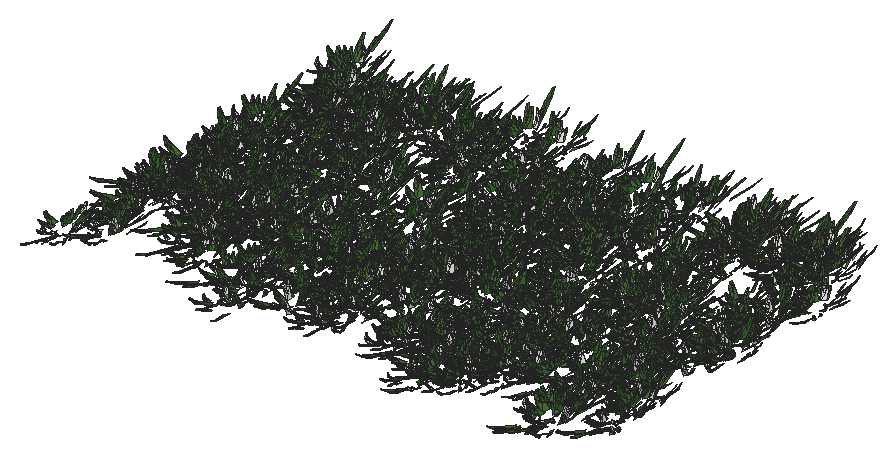
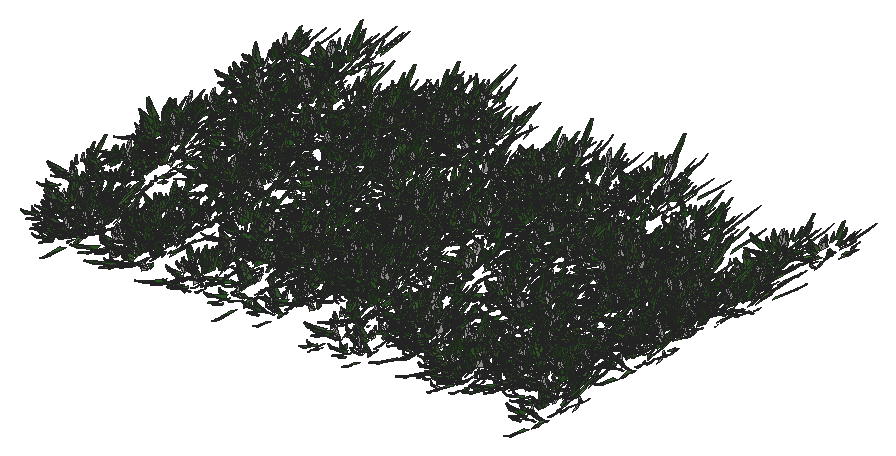
# SketchUp Ruby script. Lengths in inches.
U = 1.inch
M = Sketchup.active_model
def pt(a) = Geom::Point3d.new(a.map { |v| v * U })
def face(e, loops, mat)
  f = e.add_face(loops[0].map { |a| pt(a) })
  loops[1..].each { |l| e.add_face(l.map { |a| pt(a) }).erase! }
  f.material = f.back_material = mat if mat
  f
end
# faces: each face lists its corners as indices into pts; further lists are holes
def faces(e, pts, list, mat = nil) = list.each { |f| face(e, (f[0].is_a?(Array) ? f : [f]).map { |l| l.map { |i| pts[i] } }, mat) }
# xy, xz, yz: faces in a plane at the given z, y or x. An outline is a flat list of corners, or four numbers for a rectangle; further outlines are holes
def ring(l) = l.size == 4 ? [[l[0], l[1]], [l[2], l[1]], [l[2], l[3]], [l[0], l[3]]] : l.each_slice(2).to_a
def flat(e, list, mat, &to3) = list.each { |f| face(e, (f[0].is_a?(Array) ? f : [f]).map { |l| ring(l).map { |u, v| to3.(u, v) } }, mat) }
def xy(e, z, list, mat = nil) = flat(e, list, mat) { |x, y| [x, y, z] }
def xz(e, y, list, mat = nil) = flat(e, list, mat) { |x, z| [x, y, z] }
def yz(e, x, list, mat = nil) = flat(e, list, mat) { |y, z| [x, y, z] }
def lines(e, pts, list) = list.each { |a, b| e.add_line(pt(pts[a]), pt(pts[b])) }
# prism: a flat outline (further loops are holes) pulled along v
def prism(e, loops, v, mat = nil)
  f = face(e, loops, mat); d = Geom::Vector3d.new(v.map { |x| x * U })
  f.pushpull(f.normal.samedirection?(d) ? d.length : -d.length)
end
def box(e, o, s, mat = nil) = prism(e, [[o, [o[0] + s[0], o[1], o[2]], [o[0] + s[0], o[1] + s[1], o[2]], [o[0], o[1] + s[1], o[2]]]], [0, 0, s[2]], mat)
def at(x, y, z, deg = 0) = Geom::Transformation.translation(pt([x, y, z])) * Geom::Transformation.rotation(ORIGIN, Z_AXIS, deg.degrees)
def axes(o, x, y, z) = Geom::Transformation.new([*x, 0, *y, 0, *z, 0, *pt(o).to_a, 1])
def part(name) = M.definitions.add(name)
# library, detail: a bought-in or finely detailed component or shape, given as its bounding box
def library(name, o, s) = part(name).tap { |d| box(d.entities, o, s) }
def detail(e, o, s) = box(e.add_group.entities, o, s)
def put(e, d, t, mat = nil) = e.add_instance(d, t).tap { |i| i.material = mat if mat }
def group(e, t, mat = nil) = e.add_group.tap { |g| g.transformation = t; g.material = mat if mat }.entities
root = M.entities
M.materials.add("Material10").color = [48, 90, 38]
M.materials.add("Material11").color = [68, 110, 48]
M.materials.add("Material12").color = [48, 90, 48]
M.materials.add("Material13").color = [58, 110, 58]
M.materials.add("Material14").color = [58, 90, 38]
M.materials.add("Material15").color = [68, 100, 58]
M.materials.add("Material16").color = [48, 100, 38]
M.materials.add("Material9").color = [68, 110, 58]
c1 = part("grass00")
p = [[-0.6875,0.15,0],[-0.56,0.08,5.52],[-0.04,0.03,2.76],[0.48,-0.02,0],[0.35,-0.02,5.52],[-0.1,-0.14,5.52],
  [-0.12,0.65,8.37],[-0.42,0.65,8.37]]
faces(c1.entities,p,[[0,1,2,3],[3,2,4],[1,5,2],[5,4,2],[1,6,5],[4,5,6],[7,6,1]])
c2 = part("Group16\#1")
put(c2.entities,c1,axes([1.44,-0.61,-0.01],[0.05352,0.12609,0],[-0.10704,0.04543,0.07239],[0.06664,-0.02828,0.11628]),"Material12")
put(c2.entities,c1,axes([0.76,-0.15,-0.01],[0.04676,0.24062,0],[-0.23162,0.04501,0.06642],[0.0652,-0.01267,0.23595]),"Material9")
put(c2.entities,c1,axes([0.79,0.01,-0.01],[-0.00606,0.34651,0],[-0.34381,-0.00602,0.0432],[0.04319,0.00076,0.34386]))
put(c2.entities,c1,axes([1,0.23,-0.01],[-0.07192,0.31144,0],[-0.28722,-0.06632,0.1236],[0.12043,0.02781,0.29478]),"Material11")
put(c2.entities,c1,axes([1.66,0.77,-0.01],[-0.13828,0.29651,0],[-0.21551,-0.1005,0.22471],[0.20365,0.09498,0.23779]),"Material16")
put(c2.entities,c1,axes([0.6875,0.52,-0.01],[-0.18126,0.24051,0],[-0.22746,-0.17142,0.09788],[0.07817,0.05891,0.28481]),"Material11")
put(c2.entities,c1,axes([0.68,0.78,-0.01],[-0.215,0.18688,0],[-0.12385,-0.14248,0.21334],[0.13995,0.16101,0.18878]),"Material9")
put(c2.entities,c1,axes([0.56,1,-0.01],[-0.13756,0.07624,0],[-0.06159,-0.11112,0.0927],[0.04494,0.08108,0.12705]),"Material11")
put(c2.entities,c1,axes([0.2,0.64,-0.01],[-0.23729,0.07254,0],[-0.05711,-0.18681,0.153],[0.04473,0.14632,0.19535]),"Material16")
put(c2.entities,c1,axes([0.0625,0.72,-0.01],[-0.28874,0.02525,0],[-0.02179,-0.24916,0.14647],[0.01276,0.14591,0.25012]),"Material9")
put(c2.entities,c1,axes([-0.08,0.62,-0.01],[-0.34089,-0.04187,0],[0.03255,-0.26504,0.216],[-0.02633,0.21439,0.26703]),"Material16")
put(c2.entities,c1,axes([-0.34,0.98,-0.01],[-0.14314,-0.0493,0],[0.04397,-0.12769,0.06843],[-0.02228,0.0647,0.13505]),"Material16")
put(c2.entities,c1,axes([-0.87,1.45,-0.01],[-0.23488,-0.14114,0],[0.13761,-0.22901,0.06087],[-0.03135,0.05217,0.26717]))
put(c2.entities,c1,axes([-0.72,0.77,-0.01],[-0.14208,-0.13251,0],[0.07209,-0.0773,0.16301],[-0.11118,0.11922,0.1057]),"Material16")
put(c2.entities,c1,axes([-0.62,0.43,-0.01],[-0.14845,-0.21203,0],[0.18654,-0.13061,0.12304],[-0.10079,0.07057,0.22772]),"Material9")
put(c2.entities,c1,axes([-0.68,0.29,-0.01],[-0.13639,-0.32136,0],[0.31723,-0.13464,0.05579],[-0.05136,0.0218,0.34462]),"Material10")
put(c2.entities,c1,axes([-0.64,0.125,-0.01],[-0.0458,-0.23569,0],[0.22124,-0.043,0.08276],[-0.08124,0.01579,0.22538]),"Material13")
put(c2.entities,c1,axes([-1.6,-0.03,-0.01],[0.00576,-0.32897,0],[0.27526,0.00482,0.18018],[-0.18015,-0.00315,0.2753]),"Material11")
put(c2.entities,c1,axes([-1.36,-0.31,-0.01],[0.05718,-0.24765,0],[0.18172,0.04196,0.17267],[-0.16825,-0.03885,0.1865]),"Material16")
put(c2.entities,c1,axes([-1.54,-0.72,-0.01],[0.06537,-0.14017,0],[0.13555,0.06321,0.03939],[-0.0357,-0.01665,0.14956]))
put(c2.entities,c1,axes([-1.19,-0.9,-0.01],[0.09597,-0.12735,0],[0.11214,0.08451,0.07557],[-0.06035,-0.04548,0.14042]),"Material15")
put(c2.entities,c1,axes([-0.47,-0.54,-0.01],[0.11588,-0.10072,0],[0.0618,0.0711,0.12124],[-0.07953,-0.0915,0.0942]))
put(c2.entities,c1,axes([-0.47,-0.84,-0.01],[0.11927,-0.0661,0],[0.06603,0.11913,0.00646],[-0.00313,-0.00565,0.13621]),"Material11")
put(c2.entities,c1,axes([-0.38,-1.24,-0.01],[0.28037,-0.08571,0],[0.0618,0.20215,0.20315],[-0.05939,-0.19428,0.21139]),"Material15")
put(c2.entities,c1,axes([-0.06,-0.66,-0.01],[0.22719,-0.01987,0],[0.01247,0.14255,0.17758],[-0.01547,-0.17691,0.1431]),"Material14")
put(c2.entities,c1,axes([0.11,-0.89,-0.01],[0.14882,0.01828,0],[-0.01058,0.08611,0.12229],[0.01491,-0.12138,0.08676]),"Material12")
put(c2.entities,c1,axes([0.25,-0.72,-0.01],[0.20481,0.07053,0],[-0.06206,0.18022,0.10291],[0.03351,-0.0973,0.1906]),"Material12")
put(c2.entities,c1,axes([0.85,-1.42,-0.01],[0.16481,0.09904,0],[-0.09472,0.15762,0.05616],[0.02893,-0.04814,0.18389]),"Material11")
put(c2.entities,c1,axes([1.01,-1.09,-0.01],[0.21858,0.20385,0],[-0.17495,0.1876,0.15339],[0.10462,-0.11218,0.25652]),"Material16")
put(c2.entities,c1,axes([1.01,-0.71,-0.01],[0.08733,0.12473,0],[-0.06445,0.04512,0.13037],[0.1068,-0.07477,0.07867]),"Material12")
c3 = part("Group15\#1")
put(c3.entities,c2,at(0,0,0))
c4 = part("3darcstudiotree_grass00\#1")
put(c4.entities,c3,at(0,0,0))
put(root,c4,axes([800.04,262.41,12.99],[2.7,0,0],[0,6.17186,0],[0,0,1]))
put(root,c4,axes([917.3,263.62,12.99],[2.38747,-5.84405,0],[1.86441,3.9799,-0.01281],[0.0419,0.08945,1.56626]))
put(root,c4,axes([963.49,263.61,12.99],[3.1855,-0.69888,0],[0.31577,7.52063,-0.01064],[0.00398,0.0948,1.77558]))
put(root,c4,axes([857.27,263.68,12.99],[0.83355,-7.41561,0],[3.09264,1.81642,-0.01129],[0.04659,0.02737,1.86628]))
put(root,c4,axes([923.31,262.57,12.99],[0.33488,7.26637,0],[-2.49247,0.60022,-0.01763],[-0.08203,0.01975,1.60818]))
put(root,c4,axes([959.86,263.95,12.99],[1.44327,6.89971,0],[-2.84,3.10412,-0.01048],[-0.03086,0.03373,1.40926]))
put(root,c4,axes([930.6875,263.82,12.99],[-1.38125,4.89434,0],[-2.32777,-3.43262,-0.00439],[-0.01618,-0.02386,1.66469]))
put(root,c4,axes([809.18,269.67,12.99],[2.32785,-1.7688,0],[0.90077,6.19434,-0.00205],[0.00297,0.0204,1.79239]))
put(root,c4,axes([927.87,269.13,12.99],[1.92436,4.50414,0],[-1.90906,4.26186,-0.01838],[-0.05956,0.13295,1.65818]))
put(root,c4,axes([881,271.05,12.99],[1.20789,-7.06216,0],[2.40185,2.14654,-0.00888],[0.04378,0.03913,1.87213]))
put(root,c4,axes([917.85,271.49,12.99],[2.32526,-3.29254,0],[1.36916,5.0524,-0.00486],[0.01024,0.03779,1.42853]))
put(root,c4,axes([904.81,269.45,12.99],[-0.10545,5.83441,0],[-3.03207,-0.28635,-0.00296],[-0.01053,-0.00099,1.47961]))
put(root,c4,axes([848.52,270.28,12.99],[-2.86781,-2.90219,0],[1.05587,-5.45181,-0.0129],[0.01926,-0.09946,1.31952]))
put(root,c4,axes([870.9,270,12.99],[-2.52758,-1.38361,0],[0.5978,-5.70627,-0.00326],[0.00418,-0.03989,1.93944]))
put(root,c4,axes([857.84,271.55,12.99],[2.23594,4.22907,0],[-2.10254,5.80848,-0.00662],[-0.01529,0.04223,1.63949]))
put(root,c4,axes([975.87,271.71,12.99],[-2.17015,-3.00979,0],[1.54385,-5.81652,-0.00574],[0.00982,-0.03699,1.3472]))
put(root,c4,axes([886.64,271.69,12.99],[-3.01605,-0.65305,0],[0.2537,-6.12235,-0.02721],[0.00917,-0.22119,1.31849]))
put(root,c4,axes([930.11,272.08,12.99],[-0.07823,6.60785,0],[-2.80866,-0.17375,-0.00627],[-0.0264,-0.00163,1.62459]))
put(root,c4,axes([837.41,273.87,12.99],[2.08169,2.96658,0],[-1.3434,4.92572,-0.0044],[-0.00874,0.03206,1.30779]))
put(root,c4,axes([908.97,273.63,12.99],[-1.89759,-3.75446,0],[2.03916,-5.38532,-0.00422],[0.0086,-0.02272,1.33295]))
put(root,c4,axes([937.6,272.88,12.99],[-2.04959,5.39493,0],[-1.93192,-3.83508,-0.01448],[-0.04359,-0.08654,1.39954]))
put(root,c4,axes([905.67,278.18,12.99],[2.72294,1.91373,0],[-0.9507,7.06818,-0.02064],[-0.0201,0.1494,1.46981]))
put(root,c4,axes([829.02,279.77,12.99],[3.08767,-0.14916,0],[0.073,7.89587,-0.00824],[0.00059,0.06356,1.59977]))
put(root,c4,axes([958.97,279.01,12.99],[2.42942,0.9007,0],[-0.3986,5.61781,-0.01255],[-0.00963,0.13565,1.63564]))
put(root,c4,axes([918.12,279.84,12.99],[1.13155,-6.43414,0],[3.10428,2.85266,-0.01772],[0.06404,0.05885,1.7874]))
put(root,c4,axes([880.3125,277.63,12.99],[-0.75225,6.31697,0],[-3.37261,-2.09857,-0.0223],[-0.07136,-0.0444,1.58974]))
put(root,c4,axes([962.21,281.1,12.99],[2.38111,-3.79736,0],[1.53061,5.01498,-0.00731],[0.02053,0.06727,1.80073]))
put(root,c4,axes([849.95,278.59,12.99],[0.34869,6.4109,0],[-2.60714,0.74096,-0.00588],[-0.02211,0.00628,1.36568]))
put(root,c4,axes([885.77,281.27,12.99],[0.7386,-7.32123,0],[2.79869,1.47532,-0.00305],[0.01335,0.00704,1.76865]))
put(root,c4,axes([935.57,282.06,12.99],[2.75603,-0.4722,0],[0.25779,7.86192,-0.00347],[0.00106,0.03225,1.92949]))
put(root,c4,axes([910.36,280.67,12.99],[-1.15582,-5.1991,0],[2.69556,-3.13124,-0.00876],[0.02742,-0.03185,1.45672]))
put(root,c4,axes([942.89,280.23,12.99],[-2.27003,3.99727,0],[-1.65257,-4.9038,-0.00087],[-0.0024,-0.00712,1.68429]))
put(root,c4,axes([948.56,280.99,12.99],[-0.12493,7.61806,0],[-3.19755,-0.27399,-0.00219],[-0.00695,-0.0006,1.39308]))
put(root,c4,axes([975.82,281.26,12.99],[0.2055,7.05815,0],[-2.85108,0.43374,-0.01024],[-0.04748,0.00722,1.82096]))
put(root,c4,axes([931.78,281.15,12.99],[-2.67022,3.47951,0],[-1.66016,-6.65707,-0.01918],[-0.03722,-0.14925,1.80194]))
put(root,c4,axes([832.71,281.82,12.99],[-0.53511,7.34039,0],[-2.42448,-0.92353,-0.00349],[-0.01382,-0.00526,1.35435]))
put(root,c4,axes([860.4,282.61,12.99],[0.72731,6.87217,0],[-3.18797,1.76298,-0.01063],[-0.03416,0.01889,1.48723]))
put(root,c4,axes([896.94,284.16,12.99],[1.87008,4.14786,0],[-1.74039,4.10002,-0.00683],[-0.02423,0.05708,1.74693]))
put(root,c4,axes([923.78,283.13,12.99],[-2.48601,3.66419,0],[-1.4306,-5.07163,-0.01497],[-0.03275,-0.1161,1.4615]))
put(root,c4,axes([807.91,283.51,12.99],[-2.35772,1.35875,0],[-0.81657,-7.40372,-0.01943],[-0.01386,-0.12571,1.33771]))
put(root,c4,axes([874.16,286.77,12.99],[-0.61646,-6.32739,0],[2.39607,-1.2198,-0.00779],[0.03137,-0.01597,1.38852]))
put(root,c4,axes([877.7,287.98,12.99],[0.64081,-7.01541,0],[3.23891,1.5459,-0.01659],[0.05554,0.02651,1.55232]))
put(root,c4,axes([934.12,286.84,12.99],[-2.22659,-5.00524,0],[1.72181,-4.00226,-0.00764],[0.02885,-0.06706,1.81511]))
put(root,c4,axes([970.36,288.42,12.99],[2.84331,-3.25189,0],[1.12434,5.13679,-0.01525],[0.03164,0.14454,1.59832]))
put(root,c4,axes([866.375,287.55,12.99],[2.09267,4.86523,0],[-2.41334,5.424,-0.00938],[-0.02819,0.06335,1.95578]))
put(root,c4,axes([860.99,287.44,12.99],[1.71454,5.32814,0],[-2.62121,4.40736,-0.02079],[-0.05084,0.08548,1.35493]))
put(root,c4,axes([832.58,287.21,12.99],[-2.92579,-1.11429,0],[0.42132,-5.78045,-0.01531],[0.01289,-0.17687,1.80136]))
put(root,c4,axes([954.84,288.45,12.99],[2.5236,5.2118,0],[-1.70252,4.30755,-0.00582],[-0.01752,0.04433,1.56404]))
put(root,c4,axes([881.48,287.16,12.99],[-1.22954,6.26972,0],[-3.05141,-3.12679,-0.00369],[-0.01159,-0.01187,1.57624]))
put(root,c4,axes([804.26,288.01,12.99],[-2.71738,0.38743,0],[-0.21027,-7.70598,-0.0193],[-0.00346,-0.12694,1.33558]))
put(root,c4,axes([822.86,289.17,12.99],[-2.58469,-3.57399,0],[1.81595,-6.86221,-0.00291],[0.00482,-0.01821,1.54121]))
put(root,c4,axes([892.49,290.6,12.99],[-2.06789,-3.5248,0],[1.77407,-5.43836,-0.00029],[0.00072,-0.00221,1.69542]))
put(root,c4,axes([962.21,293.48,12.99],[2.12983,-3.59469,0],[1.82781,5.65873,-0.02283],[0.04662,0.14433,1.4512]))
put(root,c4,axes([915.64,293.58,12.99],[-2.48939,1.64634,0],[-0.90667,-7.16359,-0.00573],[-0.00569,-0.04497,1.59925]))
put(root,c4,axes([849.78,296.35,12.99],[3.03864,2.23289,0],[-0.83228,5.91815,-0.00634],[-0.00906,0.06441,1.74238]))
put(root,c4,axes([840.73,297.52,12.99],[1.03012,-7.4017,0],[3.23958,2.35585,-0.00448],[0.01639,0.01192,1.79011]))
put(root,c4,axes([837.5,297.42,12.99],[2.43111,3.00661,0],[-1.55779,6.58177,-0.00222],[-0.00378,0.01596,1.6055]))
put(root,c4,axes([942.25,297.23,12.99],[2.57694,4.09984,0],[-1.65293,5.42872,-0.01513],[-0.03119,0.10243,1.43215]))
put(root,c4,axes([821.38,299.23,12.99],[1.07572,-5.84235,0],[2.48393,2.38976,-0.00467],[0.01652,0.01589,1.41828]))
put(root,c4,axes([927.02,299.19,12.99],[0.86437,-6.35811,0],[2.8703,2.03893,-0.02169],[0.07747,0.05503,1.54236]))
put(root,c4,axes([966.95,296.75,12.99],[-2.417,-2.20097,0],[1.23575,-7.09086,-0.00121],[0.00188,-0.01079,1.92636]))
put(root,c4,axes([960.58,300.01,12.99],[2.78311,-1.49092,0],[0.79705,7.77445,-0.02268],[0.0167,0.16291,1.5468]))
put(root,c4,axes([803.91,296.6,12.99],[-1.85614,4.7772,0],[-2.25295,-4.57397,-0.01682],[-0.04757,-0.09658,1.56312]))
put(root,c4,axes([800.78,298.2,12.99],[-3.39513,-1.95103,0],[0.6221,-5.65666,-0.02201],[0.02063,-0.18756,1.34565]))
put(root,c4,axes([844.1875,300.62,12.99],[0.42428,-7.25386,0],[3.26573,0.99808,-0.0102],[0.03957,0.01209,1.76846]))
put(root,c4,axes([869.55,300.12,12.99],[-0.38453,-6.31098,0],[2.66942,-0.84987,-0.01078],[0.05195,-0.01654,1.79898]))
put(root,c4,axes([823.7,298.59,12.99],[0.52039,6.35,0],[-3.21501,1.37671,-0.00799],[-0.02639,0.0113,1.50733]))
put(root,c4,axes([816.67,298.56,12.99],[-1.20671,7.00574,0],[-2.5747,-2.3173,-0.00571],[-0.02552,-0.02297,1.8245]))
put(root,c4,axes([939.32,298.34,12.99],[-2.52179,3.319,0],[-1.73482,-6.8875,-0.0199],[-0.03481,-0.13822,1.67187]))
put(root,c4,axes([832.82,302.06,12.99],[2.17019,-5.0615,0],[2.038,4.5659,-0.0131],[0.04299,0.09632,1.79861]))
put(root,c4,axes([872.15,299.41,12.99],[-0.72304,6.51011,0],[-2.8107,-1.63115,-0.01715],[-0.061,-0.0354,1.46021]))
put(root,c4,axes([946.49,302.58,12.99],[0.31883,-7.14557,0],[2.92003,0.6808,-0.00761],[0.0365,0.00851,1.94156]))
put(root,c4,axes([807.33,299.89,12.99],[-3.25155,-0.36081,0],[0.16309,-7.67994,-0.01036],[0.00152,-0.07171,1.39846]))
put(root,c4,axes([930.53,303.07,12.99],[0.15852,-7.06641,0],[2.67457,0.31351,-0.01161],[0.04564,0.00535,1.44612]))
put(root,c4,axes([852.04,300.82,12.99],[-2.59908,2.50883,0],[-1.30475,-7.06283,-0.01449],[-0.02018,-0.10921,1.64714]))
put(root,c4,axes([878.57,302.51,12.99],[1.97562,5.89767,0],[-2.42977,4.25298,-0.02004],[-0.05173,0.09056,1.3651]))
put(root,c4,axes([909.24,302.49,12.99],[1.5456,5.93648,0],[-2.54028,3.45586,-0.00188],[-0.0075,0.01021,1.87843]))
put(root,c4,axes([923.3,303.05,12.99],[-1.79443,-4.99456,0],[2.00974,-3.77289,-0.021],[0.06382,-0.11982,1.40308]))
put(root,c4,axes([859.74,303.09,12.99],[-2.02561,-3.51282,0],[1.54104,-4.64322,-0.01586],[0.04171,-0.12567,1.52204]))
put(root,c4,axes([864.36,301.8,12.99],[-1.83508,5.30373,0],[-1.98024,-3.58012,-0.01059],[-0.03213,-0.05808,1.33934]))
put(root,c4,axes([895.01,301.85,12.99],[-2.19701,4.95047,0],[-2.33123,-5.40599,-0.01243],[-0.03382,-0.07843,1.76595]))
put(root,c4,axes([832.47,305.51,12.99],[0.69474,-6.92422,0],[2.54124,1.3323,-0.013],[0.06964,0.03651,1.96601]))
put(root,c4,axes([810.88,306.875,12.99],[1.4124,-5.84324,0],[2.17134,2.74244,-0.00396],[0.01979,0.025,1.94458]))
put(root,c4,axes([924.08,306.78,12.99],[2.8247,4.73688,0],[-1.75886,5.48043,-0.00415],[-0.00798,0.02486,1.32509]))
put(root,c4,axes([958.39,307.92,12.99],[0.18918,-5.93725,0],[2.46344,0.41016,-0.00937],[0.05346,0.0089,1.93766]))
put(root,c4,axes([943.66,307.45,12.99],[-0.98178,-5.4385,0],[3.04457,-2.87189,-0.01762],[0.05342,-0.05039,1.48208]))
put(root,c4,axes([889.55,307.28,12.99],[2.53566,4.2535,0],[-1.4585,4.54314,-0.01519],[-0.03587,0.11174,1.34969]))
put(root,c4,axes([825.69,307.64,12.99],[-2.2701,-5.60069,0],[2.40685,-5.0975,-0.02123],[0.0498,-0.10548,1.43939]))
put(root,c4,axes([930.18,307.26,12.99],[-2.36351,-2.23042,0],[0.9748,-5.3975,-0.01181],[0.0223,-0.12346,1.73426]))
put(root,c4,axes([821.16,306.41,12.99],[-2.92117,0.05351,0],[-0.02548,-7.26875,-0.00779],[-0.00024,-0.06979,1.71052]))
put(root,c4,axes([878.84,309.875,12.99],[2.04745,-6.51457,0],[2.11012,3.46529,-0.0087],[0.03185,0.0523,1.60603]))
put(root,c4,axes([914.72,307.3,12.99],[-2.93231,-1.1271,0],[0.47714,-6.48628,-0.0114],[0.00945,-0.12852,1.97478]))
put(root,c4,axes([880.41,307.71,12.99],[-3.04145,2.20175,0],[-0.83651,-6.03796,-0.01419],[-0.01972,-0.14237,1.75006]))
put(root,c4,axes([954.95,310.73,12.99],[2.62032,1.70998,0],[-0.88973,7.12409,-0.00872],[-0.00816,0.06535,1.51538]))
put(root,c4,axes([898.8,311.28,12.99],[0.93532,-6.17742,0],[2.31038,1.82785,-0.00044],[0.00165,0.00131,1.32507]))
put(root,c4,axes([892.47,309.53,12.99],[1.93534,5.53987,0],[-1.92573,3.51525,-0.01421],[-0.04631,0.08453,1.40932]))
put(root,c4,axes([839.58,307.94,12.99],[-2.73946,3.39326,0],[-1.63174,-6.88341,-0.0133],[-0.02626,-0.11077,1.94738]))
put(root,c4,axes([903.11,308.83,12.99],[-2.55398,0.81074,0],[-0.4474,-7.36433,-0.02154],[-0.00952,-0.15675,1.4342]))
put(root,c4,axes([808.54,311.97,12.99],[0.7552,-6.08854,0],[2.38927,1.54853,-0.01712],[0.0682,0.0442,1.41054]))
put(root,c4,axes([803.77,311.92,12.99],[3.3266,0.63895,0],[-0.23828,6.48218,-0.00911],[-0.00381,0.10354,1.94776]))
put(root,c4,axes([972.21,310.24,12.99],[-3.08545,-0.82643,0],[0.29814,-5.8162,-0.00847],[0.00513,-0.09999,1.82708]))
put(root,c4,axes([851.83,311.58,12.99],[-3.08185,-0.89983,0],[0.3691,-6.60553,-0.0157],[0.0096,-0.17185,1.92971]))
put(root,c4,axes([898.52,316.46,12.99],[2.51781,1.40451,0],[-0.60275,5.64605,-0.01459],[-0.01741,0.16312,1.75568]))
put(root,c4,axes([857.03,317.29,12.99],[0.97248,-5.43024,0],[2.74843,2.57188,-0.00546],[0.01653,0.01547,1.33158]))
put(root,c4,axes([820.46,317.02,12.99],[-0.67912,-5.50704,0],[3.32319,-2.14134,-0.01485],[0.05445,-0.03509,1.80381]))
put(root,c4,axes([902.66,315.91,12.99],[0.99029,6.51274,0],[-2.34145,1.86032,-0.01128],[-0.057,0.04529,1.81963]))
put(root,c4,axes([955.89,316.01,12.99],[-3.28824,0.13443,0],[-0.05478,-7.00185,-0.01042],[-0.00081,-0.10317,1.82123]))
put(root,c4,axes([882.99,319.04,12.99],[0.62571,-7.4238,0],[2.94441,1.29673,-0.00212],[0.0084,0.0037,1.6588]))
put(root,c4,axes([892.45,318,12.99],[-2.53583,-4.0256,0],[1.48452,-4.88632,-0.00375],[0.01093,-0.03599,1.82358]))
put(root,c4,axes([868.75,320.79,12.99],[2.77706,0.31623,0],[-0.16258,7.46024,-0.00527],[-0.00093,0.04278,1.59512]))
put(root,c4,axes([888.66,318.73,12.99],[0.80267,7.165,0],[-3.15194,1.84504,-0.00469],[-0.01633,0.00956,1.60422]))
put(root,c4,axes([977.2,318.72,12.99],[-2.91667,0.89835,0],[-0.39992,-6.78455,-0.01091],[-0.00661,-0.11222,1.8656]))
put(root,c4,axes([829.32,318.99,12.99],[-2.18033,3.33173,0],[-1.37245,-4.69302,-0.00767],[-0.02058,-0.07038,1.63569]))
put(root,c4,axes([805.42,320.86,12.99],[1.14348,5.78612,0],[-2.65712,2.74382,-0.01637],[-0.05127,0.05294,1.37485]))
put(root,c4,axes([942.13,321.15,12.99],[1.19769,4.92215,0],[-2.15095,2.7348,-0.00131],[-0.00659,0.00838,1.9458]))
put(root,c4,axes([810.95,320.35,12.99],[-2.92732,3.88004,0],[-1.36061,-5.36382,-0.01457],[-0.02627,-0.10357,1.33777]))
put(root,c4,axes([898.36,324.18,12.99],[0.03291,-6.00432,0],[2.63901,0.07558,-0.00992],[0.0362,0.00104,1.32167]))
put(root,c4,axes([923.375,321.65,12.99],[-3.18224,0.86052,0],[-0.37285,-7.20456,-0.02284],[-0.00893,-0.17251,1.44864]))
put(root,c4,axes([812.33,325.94,12.99],[3.02492,0.43164,0],[-0.19956,7.30757,-0.00965],[-0.00215,0.07872,1.57035]))
put(root,c4,axes([915.71,325.16,12.99],[-1.84468,-5.41874,0],[2.11551,-3.76307,-0.01663],[0.06746,-0.12,1.89037]))
put(root,c4,axes([974.43,325.54,12.99],[-1.74487,-6.43859,0],[2.07818,-2.9428,-0.00146],[0.0049,-0.00694,1.32424]))
put(root,c4,axes([967.55,327.01,12.99],[1.10448,-5.04762,0],[2.62608,3.00251,-0.01805],[0.06349,0.07259,1.58457]))
put(root,c4,axes([822.98,327.14,12.99],[0.73177,-6.13131,0],[2.98154,1.85938,-0.01691],[0.06168,0.03847,1.6028]))
put(root,c4,axes([952.48,327.69,12.99],[2.63854,-1.95158,0],[0.97491,6.88724,-0.01717],[0.0181,0.12789,1.48777]))
put(root,c4,axes([805.25,324.39,12.99],[-2.42706,4.93315,0],[-1.99413,-5.12641,-0.01814],[-0.05083,-0.13068,1.73642]))
put(root,c4,axes([971.81,324.9,12.99],[-2.78825,0.16165,0],[-0.07676,-6.91806,-0.00196],[-0.00018,-0.01617,1.49745]))
put(root,c4,axes([809.46,328.08,12.99],[2.95238,2.58076,0],[-1.15167,6.88427,-0.01506],[-0.01861,0.11123,1.52965]))
put(root,c4,axes([944.32,328.5,12.99],[2.61895,-0.43156,0],[0.18005,5.70926,-0.00836],[0.00346,0.10957,1.97523]))
put(root,c4,axes([837.86,328.27,12.99],[2.46316,1.62969,0],[-0.82342,6.50301,-0.02015],[-0.02259,0.17839,1.63787]))
put(root,c4,axes([852.25,328.88,12.99],[2.85427,2.32984,0],[-1.05964,6.78315,-0.00059],[-0.0008,0.00513,1.74794]))
put(root,c4,axes([938.04,326.12,12.99],[-2.27649,5.59218,0],[-2.46107,-5.23495,-0.01383],[-0.03262,-0.06938,1.48532]))
put(root,c4,axes([865.68,330.02,12.99],[2.66505,-1.9717,0],[0.98856,6.98188,-0.01611],[0.01782,0.12585,1.58139]))
put(root,c4,axes([843.36,327.72,12.99],[-2.36277,-1.95854,0],[0.89847,-5.66367,-0.00444],[0.00582,-0.03672,1.39182]))
put(root,c4,axes([936.27,327.97,12.99],[0.32715,6.23275,0],[-2.51704,0.69035,-0.01784],[-0.09179,0.02517,1.80168]))
put(root,c4,axes([917.54,328.21,12.99],[0.12673,7.92084,0],[-3.40439,0.28461,-0.0182],[-0.05632,0.00471,1.44668]))
put(root,c4,axes([948.17,330.9,12.99],[-0.57245,-6.81875,0],[2.52981,-1.10975,-0.00431],[0.01615,-0.00708,1.34772]))
put(root,c4,axes([828.03,328.59,12.99],[-1.27604,6.78841,0],[-2.45183,-2.4082,-0.02574],[-0.08568,-0.08415,1.32606]))
put(root,c4,axes([882.02,329.15,12.99],[-2.46614,5.52221,0],[-1.73214,-4.04198,-0.00183],[-0.0053,-0.01236,1.40539]))
put(root,c4,axes([889.25,333.54,12.99],[0.3601,-5.92996,0],[2.68874,0.85315,-0.0013],[0.00642,0.00204,1.85519]))
put(root,c4,axes([848.86,335.1,12.99],[1.7227,-4.93277,0],[1.96338,3.58283,-0.01018],[0.03495,0.06377,1.51436]))
put(root,c4,axes([840.65,336.51,12.99],[2.99045,1.2301,0],[-0.61695,7.83693,-0.01866],[-0.01187,0.15082,1.717]))
put(root,c4,axes([820.88,337.89,12.99],[1.96108,-4.17941,0],[2.3724,5.81667,-0.02398],[0.04727,0.11591,1.37951]))
put(root,c4,axes([898.62,337.12,12.99],[2.6618,2.65939,0],[-1.14151,5.97005,-0.01451],[-0.02379,0.1244,1.59989]))
put(root,c4,axes([893.15,338.71,12.99],[3.14408,2.86339,0],[-1.15655,6.63566,-0.01606],[-0.02146,0.12312,1.54782]))
put(root,c4,axes([812.29,339.55,12.99],[2.36646,-1.30514,0],[0.68088,6.45085,-0.01591],[0.01239,0.11741,1.32206]))
put(root,c4,axes([963.73,339.67,12.99],[0.15452,-7.31676,0],[2.87942,0.31773,-0.00402],[0.01346,0.00149,1.3243]))
put(root,c4,axes([908.89,336.77,12.99],[-1.5587,5.7507,0],[-2.63527,-3.73226,-0.01218],[-0.03887,-0.05506,1.59607]))
put(root,c4,axes([869.79,338.74,12.99],[2.07482,4.21999,0],[-1.74243,4.47641,-0.00943],[-0.02428,0.06239,1.39243]))
put(root,c4,axes([886.84,337.58,12.99],[-3.1737,-3.29185,0],[1.37061,-6.9047,-0.00153],[0.00253,-0.01274,1.82565]))
put(root,c4,axes([882.07,339.23,12.99],[-1.46898,-6.7837,0],[2.3252,-2.63096,-0.01272],[0.04402,-0.04981,1.37453]))
put(root,c4,axes([941.65,339.44,12.99],[-2.28628,-3.94548,0],[1.90127,-5.75674,-0.01411],[0.0333,-0.10083,1.69584]))
put(root,c4,axes([802.92,339.3,12.99],[0.50061,5.96674,0],[-3.2753,1.43588,-0.00068],[-0.00238,0.00104,1.62852]))
put(root,c4,axes([832.28,339.42,12.99],[-2.66433,-0.9731,0],[0.44718,-6.39768,-0.01241],[0.00663,-0.09491,1.31731]))
put(root,c4,axes([913.82,339.97,12.99],[-0.19578,6.41385,0],[-2.87596,-0.45871,-0.02357],[-0.09181,-0.01464,1.54387]))
put(root,c4,axes([890.14,343.22,12.99],[1.68322,-4.83671,0],[2.19066,3.98356,-0.01848],[0.05557,0.10106,1.47553]))
put(root,c4,axes([917.29,345.16,12.99],[3.49566,0.06001,0],[-0.02452,7.46354,-0.012],[-0.00034,0.10458,1.70791]))
put(root,c4,axes([973.2,343.66,12.99],[-2.66359,-1.21854,0],[0.51396,-5.8703,-0.00178],[0.00171,-0.01948,1.75352]))
put(root,c4,axes([835.2,345.84,12.99],[2.22706,4.15275,0],[-1.67404,4.69101,-0.0073],[-0.02463,0.06901,1.93831]))
put(root,c4,axes([901.01,345.72,12.99],[-1.69771,-4.76066,0],[2.1868,-4.07483,-0.00371],[0.01113,-0.02073,1.4993]))
put(root,c4,axes([910.53,345.84,12.99],[-2.35007,-5.79003,0],[2.33912,-4.96085,-0.01209],[0.03295,-0.06987,1.62724]))
put(root,c4,axes([878.33,348.61,12.99],[2.72934,-1.15279,0],[0.61394,7.5952,-0.01263],[0.00858,0.10609,1.73191]))
put(root,c4,axes([935.79,346.41,12.99],[1.76794,5.92176,0],[-2.05127,3.19997,-0.01403],[-0.06735,0.10506,1.97952]))
put(root,c4,axes([926.91,347.43,12.99],[-0.86338,-5.48895,0],[2.64408,-2.17316,-0.0171],[0.07488,-0.06155,1.79343]))
put(root,c4,axes([882.54,347.36,12.99],[-2.0906,-3.95834,0],[1.7834,-4.92165,-0.01497],[0.04542,-0.12535,1.82381]))
put(root,c4,axes([815.32,347.11,12.99],[-3.14661,1.58113,0],[-0.60088,-6.24844,-0.01858],[-0.01396,-0.14512,1.34303]))
put(root,c4,axes([899.43,348.13,12.99],[-0.68862,6.74614,0],[-2.69597,-1.43796,-0.02125],[-0.07325,-0.03907,1.34411]))
put(root,c4,axes([905.3,348.6,12.99],[-1.42218,4.76075,0],[-2.02511,-3.16106,-0.01899],[-0.08205,-0.12807,1.75992]))
put(root,c4,axes([859.875,348.76,12.99],[-1.36818,5.10488,0],[-2.1485,-3.00882,-0.01687],[-0.05663,-0.0793,1.36079]))
put(root,c4,axes([895.45,352.48,12.99],[3.16584,-2.74109,0],[1.051,6.3427,-0.01068],[0.01219,0.07355,1.31138]))
put(root,c4,axes([827.1,349.74,12.99],[-2.35658,-1.72331,0],[1.02238,-7.30529,-0.00535],[0.00595,-0.04252,1.67969]))
put(root,c4,axes([967.9,352.46,12.99],[1.61964,4.56144,0],[-2.02855,3.76363,-0.00448],[-0.01494,0.02772,1.5389]))
put(root,c4,axes([812.16,353.47,12.99],[-0.79065,-6.06523,0],[3.24073,-2.20741,-0.01047],[0.03816,-0.02599,1.7643]))
put(root,c4,axes([948.43,354.4375,12.99],[0.12508,-6.01234,0],[2.63708,0.28667,-0.0123],[0.05987,0.00651,1.7643]))
put(root,c4,axes([939.08,354.24,12.99],[-0.77602,-5.40137,0],[2.60189,-1.95327,-0.02104],[0.0775,-0.05818,1.45661]))
put(root,c4,axes([979.26,352.37,12.99],[-1.37239,5.25602,0],[-2.39344,-3.26549,-0.0186],[-0.06134,-0.08369,1.46845]))
put(root,c4,axes([885.12,355.48,12.99],[0.01784,-5.69087,0],[2.573,0.04215,-0.01704],[0.08673,0.00142,1.79616]))
put(root,c4,axes([827.71,352.96,12.99],[-1.59705,6.10398,0],[-2.23311,-3.05295,-0.01081],[-0.03586,-0.04903,1.38013]))
put(root,c4,axes([860.45,357.16,12.99],[1.39405,-6.89055,0],[3.16057,3.34113,-0.01],[0.03777,0.03993,1.98774]))
put(root,c4,axes([865.98,354.57,12.99],[-0.43359,5.47913,0],[-2.53599,-1.04863,-0.01415],[-0.05649,-0.02336,1.43376]))
put(root,c4,axes([824.24,357.38,12.99],[3.22965,-2.34805,0],[0.79658,5.7251,-0.00335],[0.0041,0.02946,1.45436]))
put(root,c4,axes([910.03,353.98,12.99],[-1.45836,5.68119,0],[-2.93726,-3.93978,-0.01374],[-0.03804,-0.05103,1.50009]))
put(root,c4,axes([899.18,354.47,12.99],[-3.05876,-0.9636,0],[0.42955,-7.12475,-0.00876],[0.00366,-0.06077,1.32289]))
put(root,c4,axes([888.9,356.19,12.99],[-2.97912,-2.28189,0],[0.83914,-5.72441,-0.02118],[0.03099,-0.2114,1.66873]))
put(root,c4,axes([816.91,356.52,12.99],[-3.38417,1.4978,0],[-0.65444,-7.72636,-0.01839],[-0.01116,-0.13175,1.50803]))
put(root,c4,axes([921.37,356.96,12.99],[-1.25703,6.55474,0],[-2.31382,-2.3186,-0.01229],[-0.0643,-0.06443,1.9803]))
put(root,c4,axes([851.8,358.9,12.99],[-1.17315,-5.24069,0],[2.87324,-3.36079,-0.02541],[0.0675,-0.07895,1.32108]))
put(root,c4,axes([856.18,361.75,12.99],[1.64853,-4.6628,0],[2.0701,3.82424,-0.01488],[0.04309,0.07961,1.35946]))
put(root,c4,axes([819.75,361.57,12.99],[2.43578,3.02171,0],[-1.66055,6.99426,-0.00178],[-0.00239,0.01007,1.34491]))
put(root,c4,axes([807.49,362.5,12.99],[2.07332,3.37249,0],[-1.6979,5.45422,-0.00585],[-0.01425,0.04576,1.68777]))
put(root,c4,axes([850.43,363.8125,12.99],[2.3952,-4.2223,0],[1.7141,5.08081,-0.00737],[0.01672,0.04957,1.42978]))
put(root,c4,axes([889.79,363.73,12.99],[2.97155,1.94076,0],[-0.77774,6.22233,-0.01128],[-0.01285,0.10278,1.61003]))
put(root,c4,axes([910.58,363.6875,12.99],[-1.90063,-5.46545,0],[2.46522,-4.47952,-0.01168],[0.02846,-0.05171,1.34439]))
put(root,c4,axes([873.52,362.23,12.99],[-3.17269,1.56415,0],[-0.63039,-6.68136,-0.00845],[-0.0059,-0.06254,1.35873]))
put(root,c4,axes([840.07,363.7,12.99],[-2.63573,-3.81155,0],[1.72114,-6.21897,-0.01513],[0.03295,-0.11904,1.79885]))
put(root,c4,axes([824.6,364.2,12.99],[1.02913,5.36668,0],[-2.80526,2.81089,-0.01361],[-0.04751,0.04761,1.60179]))
put(root,c4,axes([943.39,366.4,12.99],[0.39075,-6.34266,0],[3.28287,1.05677,-0.00524],[0.02249,0.00724,1.97007]))
put(root,c4,axes([811.98,363.36,12.99],[-1.39589,5.49192,0],[-2.87593,-3.81952,-0.00809],[-0.02934,-0.03896,1.91363]))
put(root,c4,axes([851.61,365.64,12.99],[1.52156,5.64055,0],[-2.24145,3.15938,-0.00763],[-0.02848,0.04015,1.58363]))
put(root,c4,axes([963.8125,365.87,12.99],[-2.58711,-2.65823,0],[0.99735,-5.07197,-0.02079],[0.04118,-0.20939,1.61237]))
put(root,c4,axes([835.24,365.85,12.99],[-2.1644,-3.68898,0],[1.8648,-5.717,-0.01853],[0.03938,-0.12074,1.52144]))
put(root,c4,axes([968.12,368.51,12.99],[1.55612,-5.22497,0],[2.44559,3.80583,-0.01892],[0.06717,0.10453,1.74337]))
put(root,c4,axes([955.63,367.27,12.99],[2.16914,3.77948,0],[-1.57637,4.72737,-0.01463],[-0.04322,0.12963,1.73802]))
put(root,c4,axes([831.79,367.52,12.99],[-1.21097,-5.83125,0],[2.58196,-2.80174,-0.00409],[0.01303,-0.01414,1.3842]))
put(root,c4,axes([939.11,366.23,12.99],[-3.37386,0.76397,0],[-0.2459,-5.67425,-0.0174],[-0.00865,-0.19959,1.72585]))
put(root,c4,axes([959.83,368.4,12.99],[3.03004,3.00415,0],[-1.14585,6.03892,-0.01845],[-0.02505,0.132,1.34771]))
put(root,c4,axes([971.98,368.31,12.99],[-0.77193,6.20096,0],[-2.40756,-1.56603,-0.00052],[-0.00245,-0.00159,1.67384]))
put(root,c4,axes([831.69,371.93,12.99],[1.75025,-5.37677,0],[2.73757,4.65639,-0.00846],[0.02023,0.03441,1.39582]))
put(root,c4,axes([947.57,372.9,12.99],[2.37876,1.4789,0],[-0.78868,6.62854,-0.02379],[-0.0227,0.19079,1.49895]))
put(root,c4,axes([840.77,371.19,12.99],[-2.46974,0.80175,0],[-0.41706,-6.71298,-0.00819],[-0.00381,-0.0613,1.3463]))
put(root,c4,axes([905,371.48,12.99],[-0.27403,7.88785,0],[-3.16021,-0.57367,-0.01448],[-0.04838,-0.00878,1.45727]))
put(root,c4,axes([922.76,373.72,12.99],[2.47465,3.1595,0],[-1.34267,5.495,-0.02091],[-0.04199,0.17183,1.55496]))
put(root,c4,axes([918.38,374.2,12.99],[-1.19475,-5.14031,0],[2.71612,-3.29869,-0.00698],[0.02759,-0.0335,1.8873]))
put(root,c4,axes([960.57,372.9,12.99],[-0.02238,7.75811,0],[-3.34121,-0.05037,-0.01347],[-0.04278,-0.00065,1.45625]))
put(root,c4,axes([937.7,375.07,12.99],[2.89556,2.51869,0],[-1.03866,6.23933,-0.01203],[-0.01719,0.10325,1.60927]))
put(root,c4,axes([893.55,373.79,12.99],[-0.07374,5.77333,0],[-3.01912,-0.20148,-0.00454],[-0.01823,-0.00122,1.66362]))
put(root,c4,axes([804.2,374.18,12.99],[0.3933,6.70447,0],[-3.21596,0.98578,-0.0098],[-0.03761,0.01153,1.72283]))
put(root,c4,axes([942.42,373.52,12.99],[-2.21963,4.26552,0],[-1.56647,-4.25929,-0.00081],[-0.00276,-0.00751,1.76997]))
put(root,c4,axes([873.28,374.71,12.99],[-2.15222,5.57282,0],[-2.12129,-4.28073,-0.01581],[-0.04065,-0.08202,1.33135]))
put(root,c4,axes([963.26,375.14,12.99],[-1.66298,5.45753,0],[-2.14442,-3.41432,-0.01437],[-0.06314,-0.10052,1.91898]))
put(root,c4,axes([862.39,375.71,12.99],[-0.44601,6.46154,0],[-2.83602,-1.02288,-0.0149],[-0.07177,-0.02589,1.9212]))
